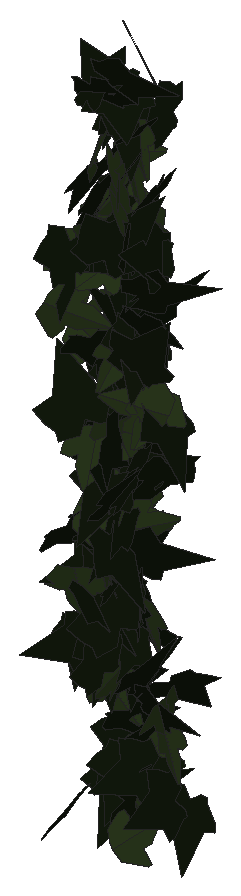
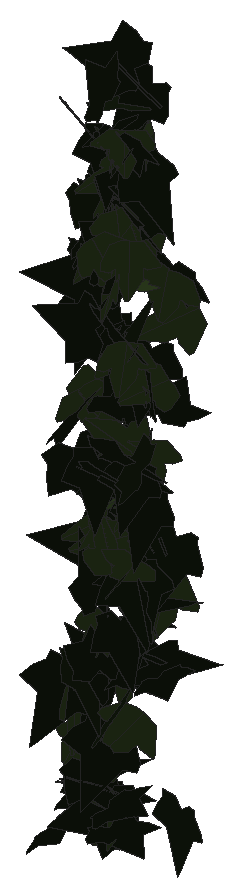
# SketchUp Ruby script. Lengths in inches.
U = 1.inch
M = Sketchup.active_model
def pt(a) = Geom::Point3d.new(a.map { |v| v * U })
def face(e, loops, mat)
  f = e.add_face(loops[0].map { |a| pt(a) })
  loops[1..].each { |l| e.add_face(l.map { |a| pt(a) }).erase! }
  f.material = f.back_material = mat if mat
  f
end
# faces: each face lists its corners as indices into pts; further lists are holes
def faces(e, pts, list, mat = nil) = list.each { |f| face(e, (f[0].is_a?(Array) ? f : [f]).map { |l| l.map { |i| pts[i] } }, mat) }
# xy, xz, yz: faces in a plane at the given z, y or x. An outline is a flat list of corners, or four numbers for a rectangle; further outlines are holes
def ring(l) = l.size == 4 ? [[l[0], l[1]], [l[2], l[1]], [l[2], l[3]], [l[0], l[3]]] : l.each_slice(2).to_a
def flat(e, list, mat, &to3) = list.each { |f| face(e, (f[0].is_a?(Array) ? f : [f]).map { |l| ring(l).map { |u, v| to3.(u, v) } }, mat) }
def xy(e, z, list, mat = nil) = flat(e, list, mat) { |x, y| [x, y, z] }
def xz(e, y, list, mat = nil) = flat(e, list, mat) { |x, z| [x, y, z] }
def yz(e, x, list, mat = nil) = flat(e, list, mat) { |y, z| [x, y, z] }
def lines(e, pts, list) = list.each { |a, b| e.add_line(pt(pts[a]), pt(pts[b])) }
# prism: a flat outline (further loops are holes) pulled along v
def prism(e, loops, v, mat = nil)
  f = face(e, loops, mat); d = Geom::Vector3d.new(v.map { |x| x * U })
  f.pushpull(f.normal.samedirection?(d) ? d.length : -d.length)
end
def box(e, o, s, mat = nil) = prism(e, [[o, [o[0] + s[0], o[1], o[2]], [o[0] + s[0], o[1] + s[1], o[2]], [o[0], o[1] + s[1], o[2]]]], [0, 0, s[2]], mat)
def at(x, y, z, deg = 0) = Geom::Transformation.translation(pt([x, y, z])) * Geom::Transformation.rotation(ORIGIN, Z_AXIS, deg.degrees)
def axes(o, x, y, z) = Geom::Transformation.new([*x, 0, *y, 0, *z, 0, *pt(o).to_a, 1])
def part(name) = M.definitions.add(name)
# library, detail: a bought-in or finely detailed component or shape, given as its bounding box
def library(name, o, s) = part(name).tap { |d| box(d.entities, o, s) }
def detail(e, o, s) = box(e.add_group.entities, o, s)
def put(e, d, t, mat = nil) = e.add_instance(d, t).tap { |i| i.material = mat if mat }
def group(e, t, mat = nil) = e.add_group.tap { |g| g.transformation = t; g.material = mat if mat }.entities
root = M.entities
M.materials.add("efeu1").color = [18, 25, 13]
M.materials.add("efeu2").color = [43, 57, 29]
c1 = part("ivyleaf_9")
p = [[1.54,2.16,1.25],[1.36,2.04,1.19],[-0.21,0.99,0.68],[-0.71,1.11,0.82],[-0.85,0.86,0.67],[-0.8,0.17,0.21],
  [-0.9,-0.01,0.1],[-0.67,-0.16,-0.02],[-0.08,-0.08,-0.05],[-0.03,-0.6,-0.4],[0.65,-0.88,-0.66],[0.83,-0.6,-0.49],
  [1.29,-0.42,-0.43],[1.8125,-0.07,-0.26],[1.21,0.44,0.15]]
faces(c1.entities,p,[[0,1,2,3,4,5,6,7,8,9,10,11,12,13,14]],"efeu1")
c2 = part("ivyleaf_10")
p = [[0,0.5,-0.03],[-0.0625,2.02,-0.43],[-0.19,2.01,-0.46],[-0.54,1.05,-0.29],[-0.52,0.625,-0.18],[-0.83,0.76,-0.28],
  [-1.16,0.64,-0.33],[-1.15,0.33,-0.24],[-0.77,-0.39,0.02],[-0.3,-0.51,0.16],[0.04,-0.48,0.23],[-0.02,2.01,-0.4375],
  [-0.06,2.01,-0.43],[0.04,-0.49,0.23],[0.67,-0.49,0.14],[1.38,0.36,-0.2],[1.375,0.51,-0.24],[0.81,0.65,-0.19],
  [0.62,0.59,-0.15],[0.6,1.09,-0.28],[0.5,1.23,-0.31]]
faces(c2.entities,p,[[0,1,2,3,4,5,6,7,8,9,10],[11,12,0,13,14,15,16,17,18,19,20]],"efeu2")
put(root,c1,axes([597.68,127.19,216.3],[-0.89912,0.12455,-0.45826],[-0.45207,0.07595,0.90763],[0.14541,1.00631,-0.01178]))
put(root,c1,axes([595.74,127.01,209.03],[-0.11047,0.92219,0.33804],[-0.03291,0.33651,-0.92876],[-0.98164,-0.11506,-0.00691]))
put(root,c1,axes([596.35,127.6,227.26],[-1.02165,-0.43663,0.11309],[0.11105,0.0279,1.1109],[-0.43716,1.02751,0.0179]))
put(root,c1,axes([597.76,127.6875,222.07],[0.49242,-0.88914,-0.4928],[-0.23519,0.43308,-1.01638],[0.989,0.54569,0.00366]))
put(root,c2,axes([598.41,127.17,238.28],[-0.48366,0.76583,0.78404],[-0.47666,0.62471,-0.90425],[-0.98692,-0.67703,0.05249]))
put(root,c1,axes([598.2,128.1,223.28],[-1.04138,0.25838,-0.48017],[0.46762,-0.10923,-1.07294],[-0.28046,-1.14154,-0.00602]))
put(root,c2,axes([595.22,127.39,232.02],[-0.49296,-0.24559,-0.99546],[0.88842,0.44907,-0.55074],[0.51183,-1.01601,-0.0028]))
put(root,c1,axes([598.91,127.73,225.35],[-0.81861,0.81752,-0.04347],[0.03076,-0.03071,-1.15692],[-0.81809,-0.81919,-0.00001]))
put(root,c1,axes([595.2,128.12,234.46],[-0.8254,-0.25972,-0.64052],[0.59825,0.23118,-0.86467],[0.34615,-1.01887,-0.03292]))
put(root,c1,axes([597.3125,128.26,224.49],[-0.97685,-0.34915,-0.27907],[0.27175,0.06858,-1.03705],[0.35487,-1.01361,0.02596]))
put(root,c2,axes([597.18,127.25,239.34],[0.40755,-0.18459,0.94141],[-0.59795,0.75097,0.40611],[-0.75019,-0.69886,0.18773]))
put(root,c1,axes([597.83,127.32,226.86],[0.30223,-0.19316,-1.04798],[-0.86631,0.58981,-0.35855],[0.62055,0.91746,0.00986]))
put(root,c1,axes([598.03,126.93,224.1],[0.48539,0.56933,0.87843],[0.37678,0.80836,-0.73211],[-0.97664,0.59482,0.15414]))
put(root,c2,axes([595.95,127.78,219.65],[-1.10034,-0.35277,-0.11717],[0.11218,0.03391,-1.15551],[0.3544,-1.10604,0.00195]))
put(root,c2,axes([598.36,127.125,238.83],[0.13889,0.08286,-1.17273],[-0.41504,1.10831,0.02916],[1.09995,0.40772,0.15908]))
put(root,c1,axes([595.875,128.66,216.43],[-0.15637,-0.3981,-0.89438],[-0.15552,-0.88412,0.42072],[-0.96655,0.20667,0.077]))
put(root,c1,axes([597.59,127.58,234.99],[-0.33919,-0.14159,1.12986],[1.11512,0.19735,0.35949],[-0.23051,1.16305,0.07655]))
put(root,c2,axes([597.18,128.79,215.42],[-0.16496,-0.0303,1.10441],[0.52657,-0.98383,0.05166],[0.97127,0.52823,0.15957]))
put(root,c2,axes([596.45,128.72,233.44],[-0.91189,-0.04908,0.28753],[0.1329,-0.91002,0.26614],[0.25966,0.2934,0.87357]))
put(root,c1,axes([596.24,127.94,219.08],[0.83632,-0.71948,-0.22246],[-0.04485,0.28428,-1.08801],[0.75175,0.81738,0.18258]))
put(root,c2,axes([597.1,127.77,221.45],[-0.91608,0.61726,0.33442],[-0.31405,0.13139,-1.1028],[-0.62787,-0.96632,0.06367]))
put(root,c1,axes([596.92,128.71,223.79],[-0.22534,0.05875,0.9695],[-0.10491,-0.9909,0.03566],[0.9656,-0.09395,0.23013]))
put(root,c1,axes([597.93,127.85,218.15],[-1.20266,-0.16025,-0.31583],[-0.30978,-0.06593,1.21306],[-0.17166,1.24169,0.02365]))
put(root,c1,axes([597.375,128.125,242.8],[0.56666,-0.21257,0.85054],[0.83158,-0.19037,-0.60161],[0.27762,1.00413,0.066]))
put(root,c2,axes([596.35,128.31,225.87],[0.91677,0.5159,-0.11245],[-0.10842,-0.0366,-1.05175],[-0.51676,0.92292,0.02116]))
put(root,c1,axes([598.56,128.3,229.91],[-0.46509,-0.10818,0.92864],[0.86566,-0.44162,0.3821],[0.35316,0.94003,0.28637]))
put(root,c1,axes([596.64,128.21,238.64],[-0.33833,1.01158,-0.43434],[0.09739,-0.42511,-1.06593],[-1.09657,-0.34987,0.03934]))
put(root,c1,axes([596.47,127.65,236.78],[-0.19258,0.95956,-0.3826],[-0.27248,0.32822,0.96034],[0.99644,0.2752,0.18866]))
put(root,c1,axes([596.5,128.03,242.24],[1.02917,0.29788,-0.18227],[-0.17223,-0.06049,-1.07137],[-0.30379,1.04344,-0.01008]))
put(root,c2,axes([597.84,128.3125,207.92],[0.62888,0.00293,-0.75281],[0.75191,0.04577,0.6283],[0.037,-0.97986,0.0271]))
put(root,c1,axes([595.46,127.73,221.85],[0.29961,1.11838,0.22488],[0.0554,0.21797,-1.15781],[-1.13942,0.30467,0.00284]))
put(root,c2,axes([595.09,128.5625,234.23],[1.15571,0.23269,0.39445],[0.38704,0.0761,-1.1789],[-0.24482,1.2188,-0.0017]))
put(root,c2,axes([598.8,129.0625,227.71],[0.26313,0.3553,1.04017],[-0.59032,-0.85654,0.44191],[0.9272,-0.64616,-0.01384]))
put(root,c2,axes([596.47,127.97,222.76],[0.30246,0.29473,1.09545],[0.69036,0.85179,-0.41978],[-0.90015,0.75229,0.04613]))
put(root,c1,axes([597.04,129.14,241.58],[-0.24246,-0.94602,-0.08289],[0.67617,-0.11191,-0.70063],[0.6668,-0.23051,0.68034]))
put(root,c2,axes([597.34,128.86,230.2],[0.4623,0.70923,-0.52342],[-0.33383,-0.40614,-0.84517],[-0.81581,0.5681,0.04923]))
put(root,c2,axes([596.57,128.67,235.16],[-0.54784,-0.94769,0.22801],[0.15063,0.1761,1.09386],[-0.96302,0.56666,0.04139]))
put(root,c1,axes([598.9,129.4,234.49],[-0.23155,-0.08125,0.98555],[-0.39713,-0.91935,-0.1691],[0.90564,-0.42392,0.17783]))
put(root,c1,axes([599.41,129.52,209.8],[-0.28324,-0.51993,0.85137],[-0.37833,-0.76292,-0.59178],[0.92305,-0.47224,0.01869]))
put(root,c1,axes([598.22,129.45,210.875],[-0.51563,-0.42462,0.73612],[-0.43315,-0.60946,-0.65497],[0.73113,-0.66054,0.13112]))
put(root,c1,axes([596.36,129.1,216.44],[0.00703,-1.02737,-0.11169],[-0.00105,0.11169,-1.02739],[1.03342,0.0071,-0.00028]))
put(root,c1,axes([596.18,128.33,230.39],[0.56264,0.81641,-0.26488],[-0.16334,-0.20909,-0.99139],[-0.84262,0.58567,0.0153]))
put(root,c1,axes([597.48,128.6,220.15],[-0.72348,0.75288,0.01056],[-0.00801,0.00695,-1.04415],[-0.75291,-0.72352,0.00096]))
put(root,c1,axes([596.87,128.23,242.11],[-0.03834,0.56451,0.88311],[-0.64167,0.68609,-0.46643],[-0.82874,-0.55734,0.32029]))
put(root,c1,axes([595.07,129.21,216.33],[-0.23892,-0.81903,-0.05977],[0.03094,0.05323,-0.85304],[0.82063,-0.24046,0.01476]))
put(root,c1,axes([595.82,129.39,219.4],[-0.60224,-0.23806,0.59769],[-0.46859,-0.39867,-0.63095],[0.44083,-0.749,0.14587]))
put(root,c1,axes([598.67,128.5,232.07],[0.94016,0.31159,-0.46753],[-0.44967,-0.12913,-0.9903],[-0.33686,1.04202,0.01708]))
put(root,c1,axes([597.95,129.375,230.85],[-0.28435,-0.98477,-0.05517],[0.01569,0.05289,-1.025],[0.98619,-0.28478,0.0004]))
put(root,c1,axes([598.1,128.58,215.12],[0.32455,0.93277,0.0583],[-0.06779,-0.03806,0.98628],[0.93213,-0.32755,0.05143]))
put(root,c1,axes([597.16,129.13,237],[-0.94182,0.16671,-0.06716],[0.06582,-0.01345,-0.95646],[-0.16724,-0.94411,0.00177]))
put(root,c1,axes([597.75,129.38,219.75],[-0.2317,-0.01286,-0.95951],[0.93157,-0.23981,-0.22174],[-0.23021,-0.95751,0.06842]))
put(root,c1,axes([596.98,129.48,216.67],[-0.77428,-0.75271,-0.1101],[0.10029,0.05473,-1.07943],[0.75408,-0.78016,0.03051]))
put(root,c1,axes([597.79,129.28,238.82],[-0.64757,0.54586,-0.58703],[0.31245,-0.52308,-0.83107],[-0.7382,-0.70025,0.1632]))
put(root,c2,axes([597.58,129.55,235.53],[-0.30579,-0.4987,0.76252],[-0.32545,-0.69147,-0.58275],[0.85101,-0.44364,0.05114]))
put(root,c1,axes([598.09,128.71,221.02],[0.60705,-0.00079,0.94576],[0.94565,0.01755,-0.60697],[-0.01434,1.12369,0.01015]))
put(root,c2,axes([596.74,128.6,219.96],[-0.76753,0.63572,0.58904],[-0.45937,0.3688,-0.99659],[-0.73491,-0.89446,0.00774]))
put(root,c2,axes([596.89,128.76,225.8125],[-0.41438,-0.5741,0.82611],[0.5852,0.58916,0.70298],[-0.81828,0.71207,0.0844]))
put(root,c1,axes([598.19,129.28,213.95],[0.55977,-0.41995,0.80627],[0.70002,-0.40498,-0.69694],[0.57999,0.89409,0.06302]))
put(root,c2,axes([598.74,129.39,227.9375],[0.59219,0.7082,-0.49333],[-0.33911,-0.35926,-0.9228],[-0.79368,0.6819,0.02619]))
put(root,c1,axes([598.43,128.62,233.07],[0.62142,0.03516,0.92551],[0.88738,0.29659,-0.60709],[-0.26525,1.0746,0.13727]))
put(root,c1,axes([597.2,129.54,240.64],[-0.15744,-0.94995,-0.15826],[0.06896,0.14883,-0.96194],[0.96057,-0.16638,0.04312]))
put(root,c1,axes([599.2,129.32,225.22],[-0.09213,0.81657,-0.76424],[-0.07078,-0.76955,-0.81371],[-1.11617,-0.0186,0.11468]))
put(root,c2,axes([597.625,129.5625,239.76],[-0.62599,0.26321,-0.69586],[0.42872,-0.61562,-0.61853],[-0.60803,-0.70505,0.2803]))
put(root,c2,axes([598.02,128.46,222.34],[-0.13162,-0.16156,-1.1183],[0.60882,0.93831,-0.20721],[0.95186,-0.62249,-0.0221]))
put(root,c1,axes([596.64,129.71,230.57],[0.51327,-0.96629,0.19404],[-0.07458,0.18007,1.094],[-0.98276,-0.51834,0.01832]))
put(root,c2,axes([596.14,129.15,224.43],[0.34312,-0.82288,0.10887],[0.78754,0.28551,-0.32402],[0.26225,0.21924,0.83059]))
put(root,c1,axes([596.64,129.42,229.64],[-0.39909,-0.22501,-0.93669],[0.87415,0.34146,-0.45447],[0.40481,-0.9592,0.05794]))
put(root,c1,axes([595.55,128.84,221.11],[0.61981,0.26266,0.56562],[0.53152,0.19461,-0.67282],[-0.32618,0.81622,-0.0216]))
put(root,c1,axes([596.99,129.76,210.71],[-0.70513,-0.60463,-0.18906],[0.15951,0.10433,-0.92855],[0.61309,-0.72255,0.02413]))
put(root,c1,axes([598.34,129.67,234.87],[-0.90444,-0.26445,-0.32395],[0.30367,0.11534,-0.942],[0.2875,-0.95376,-0.0241]))
put(root,c2,axes([597,129.42,236.72],[0.49861,0.87692,-0.15448],[-0.06817,-0.13894,-1.00872],[-0.8878,0.50316,-0.00931]))
put(root,c2,axes([597.18,129.6,209.41],[-0.29447,0.21401,-0.87107],[0.73601,-0.46637,-0.36339],[-0.51268,-0.79245,-0.02138]))
put(root,c2,axes([596.19,129.46,224.14],[-0.19789,0.93291,-0.28069],[0.03193,-0.28006,-0.95332],[-0.9737,-0.19878,0.02578]))
put(root,c1,axes([596.97,129.8125,228.67],[-0.54217,-0.73513,-0.10513],[0.05883,0.08724,-0.91343],[0.74028,-0.54533,-0.00441]))
put(root,c1,axes([596.11,130.19,240.01],[-0.18454,-0.4895,0.88906],[0.07197,-0.90767,-0.48481],[1.01235,-0.02471,0.19653]))
put(root,c1,axes([595.96,128.91,228.8],[0.23217,-0.12038,0.98571],[-0.25695,0.97053,0.17905],[-0.95921,-0.28912,0.19062]))
put(root,c1,axes([598.88,129.72,227.27],[0.31897,-1.03019,-0.15265],[-0.04754,0.14508,-1.07844],[1.04036,0.32248,-0.00247]))
put(root,c1,axes([596.67,130.24,233.75],[-0.21839,-0.40478,0.82177],[-0.40359,-0.71587,-0.45988],[0.82235,-0.45883,-0.00746]))
put(root,c1,axes([597.88,128.89,234.48],[0.07262,-0.33673,1.16286],[0.44281,1.09162,0.28845],[-1.12675,0.40731,0.18831]))
put(root,c1,axes([598.43,129.67,237.47],[-0.50007,0.74283,-0.45298],[0.19066,-0.41621,-0.89301],[-0.8489,-0.53107,0.06627]))
put(root,c2,axes([594.92,129.34,229.86],[0.55471,0.2393,0.88076],[0.7595,0.45052,-0.60075],[-0.50612,0.93834,0.06382]))
put(root,c1,axes([597.66,129.16,239.85],[0.10116,0.96642,-0.04305],[-0.00547,-0.04271,-0.9717],[-0.96736,0.1013,0.00099]))
put(root,c2,axes([597.4,129.58,237.93],[-0.38225,0.87555,-0.13351],[0.06467,-0.11744,-0.95528],[-0.88331,-0.38749,-0.01216]))
put(root,c2,axes([596,129.64,214.23],[-0.8718,-0.20298,-0.65841],[0.6826,-0.11023,-0.86985],[0.09359,-1.08691,0.21117]))
put(root,c1,axes([595.52,129.34,224.34],[0.7701,0.41199,-0.49515],[-0.45823,-0.192,-0.87243],[-0.4527,0.89519,0.04077]))
put(root,c2,axes([599.01,129.51,214.19],[-0.0454,-1.02151,-0.39808],[-0.01975,0.39912,-1.02192],[1.09616,-0.03512,-0.0349]))
put(root,c2,axes([598.77,129.98,212.47],[-0.74598,0.29817,-0.58635],[0.40045,-0.49749,-0.76246],[-0.52187,-0.80796,0.25308]))
put(root,c1,axes([598.1,130.06,225.07],[-0.95047,-0.05411,0.08269],[-0.08173,-0.01897,-0.95191],[0.05555,-0.95387,0.01424]))
put(root,c1,axes([597.33,129.8125,225.92],[-0.64834,0.23991,0.70636],[-0.67517,0.20928,-0.69079],[-0.31725,-0.93567,0.0266]))
put(root,c1,axes([597.5,129.48,231.51],[-0.48407,0.46622,0.72834],[-0.53742,0.49175,-0.67196],[-0.67751,-0.72318,0.01262]))
put(root,c1,axes([596.51,130.38,209.52],[-0.69365,-0.80276,-0.04094],[0.05959,0.00257,-1.06004],[0.80159,-0.69486,0.04337]))
put(root,c2,axes([597.77,129.73,218.08],[-0.9321,0.40462,-0.16858],[0.15255,-0.07194,-1.01612],[-0.41093,-0.94449,0.00517]))
put(root,c1,axes([597.56,128.92,209.5],[-0.0381,0.70891,-0.91126],[-0.26812,0.8814,0.69689],[1.12297,0.23449,0.13547]))
put(root,c1,axes([595.875,129.6,225.59],[0.68932,0.48732,-0.32741],[-0.27491,-0.17826,-0.84409],[-0.51875,0.74201,0.01225]))
put(root,c2,axes([597.02,129.3125,238.9],[0.03596,-0.34893,-0.93535],[0.54703,0.78983,-0.27361],[0.8351,-0.50235,0.2195]))
put(root,c1,axes([597.27,130.25,216.55],[0.94852,-0.12222,0.2382],[-0.23515,0.03888,0.95633],[-0.12799,-0.9772,0.00825]))
put(root,c1,axes([598.96,129.91,241.07],[-0.87151,0.50727,0.20358],[-0.17711,0.10041,-1.00839],[-0.51711,-0.88932,0.00227]))
put(root,c1,axes([595.67,130.42,221.53],[0.3151,-0.95114,0.23169],[0.10469,-0.20926,-1.00144],[0.97334,0.33042,0.03271]))
put(root,c2,axes([596.8,129.72,222.29],[-0.38513,-0.12615,-0.9075],[0.88136,0.21799,-0.40434],[0.25037,-0.96144,0.02739]))
put(root,c1,axes([598.75,129.59,215.78],[-0.45276,0.98097,0.11986],[-0.02172,0.12193,-1.07997],[-0.98803,-0.4522,-0.03119]))
put(root,c1,axes([597.66,129.82,225.48],[0.64615,0.47342,-0.56617],[-0.50184,-0.26992,-0.79843],[-0.54115,0.8156,0.0644]))
put(root,c1,axes([595.1,130.43,226.25],[0.61696,-0.7067,0.39551],[0.24707,-0.30925,-0.93798],[0.77124,0.6644,-0.01591]))
put(root,c1,axes([596.66,130.73,242.76],[0.25075,-0.5328,0.88166],[0.40933,-0.78117,-0.58848],[0.94534,0.47957,0.02095]))
put(root,c2,axes([595.9,130.125,235.76],[-0.78197,-0.54346,0.027],[-0.02173,-0.01605,-0.95228],[0.5437,-0.78227,0.00078]))
put(root,c2,axes([597.42,130.1,222.9],[-0.18441,0.93288,-0.10467],[0.01374,-0.10398,-0.95091],[-0.93863,-0.1848,0.00665]))
put(root,c2,axes([596.76,130.33,221.59],[-0.09213,-0.97365,-0.06234],[0.03827,-0.06618,0.97699],[-0.97489,0.08941,0.04424]))
put(root,c2,axes([597.78,129.41,234.95],[0.11465,0.23421,0.95616],[-0.25646,0.93649,-0.19864],[-0.95043,-0.22444,0.16894]))
put(root,c1,axes([598.3125,130.67,211.08],[-0.92458,-0.03522,0.32565],[-0.29819,-0.313,-0.88048],[0.13553,-0.92894,0.28432]))
put(root,c1,axes([597.15,129.62,213.08],[0.64205,0.8845,-0.01366],[-0.00761,-0.01135,-1.09296],[-0.88457,0.6421,-0.00051]))
put(root,c2,axes([597.15,130.53,235.66],[-0.55229,-0.62053,0.46142],[-0.22717,-0.41181,-0.82571],[0.73916,-0.59021,0.091]))
put(root,c1,axes([596.19,130.9,214.6875],[0.16195,-0.8234,0.56622],[0.11475,-0.55449,-0.83916],[0.99269,0.19843,0.00463]))
put(root,c2,axes([597.84,130.41,211.39],[0.74222,0.21167,-0.61145],[-0.60398,-0.10715,-0.77025],[-0.23211,0.95566,0.04906]))
put(root,c1,axes([595.86,130.61,241.27],[-0.8058,-0.34404,-0.49094],[0.48685,0.10436,-0.87222],[0.3498,-0.93778,0.08304]))
put(root,c1,axes([597.71,130.44,212.04],[-0.21094,0.68411,-0.6843],[0.02124,-0.69693,-0.70328],[-0.96738,-0.16448,0.13378]))
put(root,c2,axes([595.55,130.21,221.72],[0.7767,0.35445,0.52156],[0.4805,0.20321,-0.85367],[-0.40838,0.91324,-0.01248]))
put(root,c1,axes([595.66,129.9,221.11],[0.40973,0.81496,-0.59134],[-0.65936,-0.26533,-0.82254],[-0.76098,0.6687,0.39431]))
put(root,c2,axes([595.86,130.32,241.08],[0.76473,0.64882,0.05094],[0.03845,0.03341,-1.00288],[-0.64968,0.76569,0.0006]))
put(root,c1,axes([594.61,130.71,220.16],[0.09887,-0.09167,-1.07306],[1.07695,0.00299,0.09898],[-0.00542,-1.0776,0.09155]))
put(root,c1,axes([599.1875,129.71,215.08],[0.71618,0.80559,0.0967],[0.00965,0.12052,-1.07547],[-0.81132,0.71256,0.07257]))
put(root,c1,axes([596.01,131.08,210.95],[-0.39885,-0.85576,0.34841],[-0.16077,-0.30942,-0.94404],[0.90988,-0.4298,-0.01408]))
put(root,c2,axes([595.85,130.4,231.32],[-0.64568,-0.66081,-0.10091],[0.18355,-0.04036,-0.91018],[0.64278,-0.65227,0.15855]))
put(root,c1,axes([597.27,130.4375,219.91],[0.23305,0.76695,0.52291],[-0.19151,-0.48781,0.80083],[0.90828,-0.29964,0.03469]))
put(root,c1,axes([599.0625,131,208.98],[-0.0199,-1.0511,0.16075],[-0.03251,-0.1601,-1.05088],[1.06282,-0.02457,-0.02914]))
put(root,c1,axes([597.98,129.83,231.4375],[0.13993,0.92716,-0.37618],[-0.08,0.38899,0.92897],[0.99736,-0.09888,0.1273]))
put(root,c1,axes([596.18,130.26,218.9],[0.4408,0.45301,-0.73059],[-0.68215,-0.31529,-0.60708],[-0.52312,0.79288,0.17602]))
put(root,c2,axes([596.57,130.35,234.51],[-0.78552,0.52414,0.0251],[-0.02851,0.00249,-0.94423],[-0.52396,-0.78591,0.01375]))
